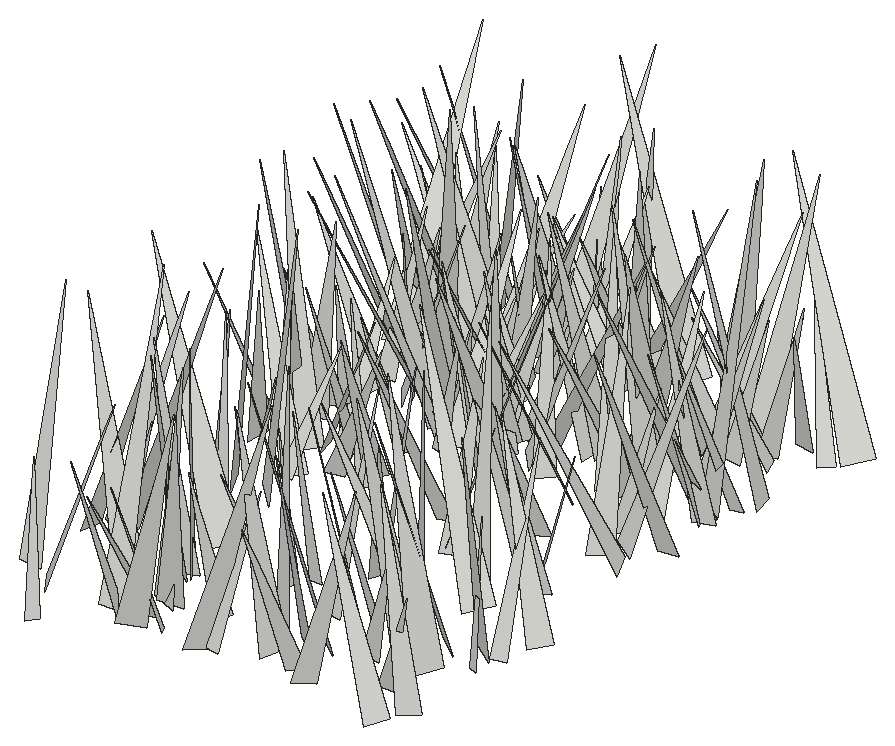
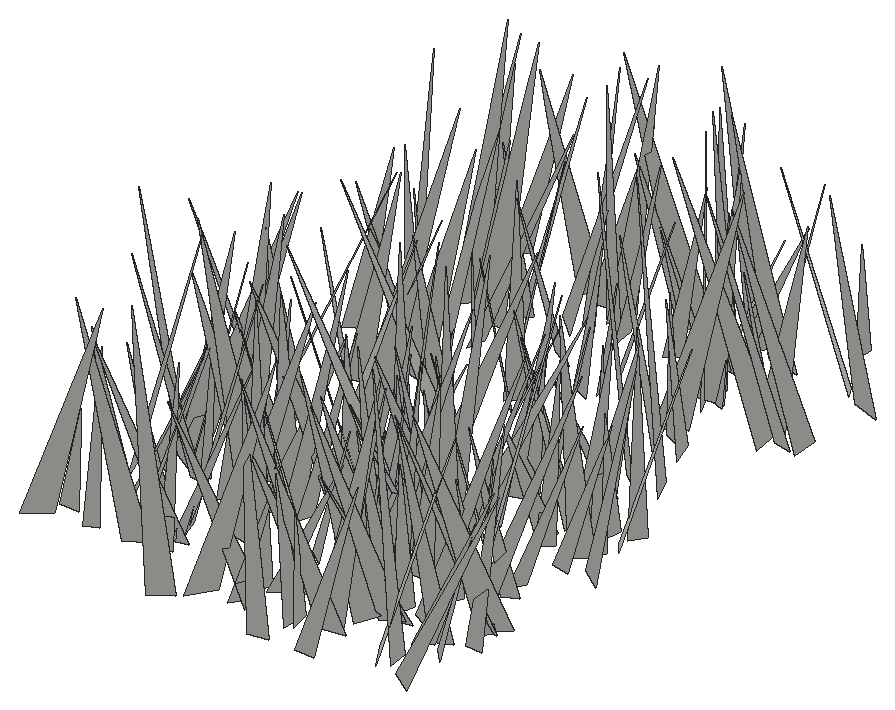
# SketchUp Ruby script. Lengths in inches.
U = 1.inch
M = Sketchup.active_model
def pt(a) = Geom::Point3d.new(a.map { |v| v * U })
def face(e, loops, mat)
  f = e.add_face(loops[0].map { |a| pt(a) })
  loops[1..].each { |l| e.add_face(l.map { |a| pt(a) }).erase! }
  f.material = f.back_material = mat if mat
  f
end
# faces: each face lists its corners as indices into pts; further lists are holes
def faces(e, pts, list, mat = nil) = list.each { |f| face(e, (f[0].is_a?(Array) ? f : [f]).map { |l| l.map { |i| pts[i] } }, mat) }
# xy, xz, yz: faces in a plane at the given z, y or x. An outline is a flat list of corners, or four numbers for a rectangle; further outlines are holes
def ring(l) = l.size == 4 ? [[l[0], l[1]], [l[2], l[1]], [l[2], l[3]], [l[0], l[3]]] : l.each_slice(2).to_a
def flat(e, list, mat, &to3) = list.each { |f| face(e, (f[0].is_a?(Array) ? f : [f]).map { |l| ring(l).map { |u, v| to3.(u, v) } }, mat) }
def xy(e, z, list, mat = nil) = flat(e, list, mat) { |x, y| [x, y, z] }
def xz(e, y, list, mat = nil) = flat(e, list, mat) { |x, z| [x, y, z] }
def yz(e, x, list, mat = nil) = flat(e, list, mat) { |y, z| [x, y, z] }
def lines(e, pts, list) = list.each { |a, b| e.add_line(pt(pts[a]), pt(pts[b])) }
# prism: a flat outline (further loops are holes) pulled along v
def prism(e, loops, v, mat = nil)
  f = face(e, loops, mat); d = Geom::Vector3d.new(v.map { |x| x * U })
  f.pushpull(f.normal.samedirection?(d) ? d.length : -d.length)
end
def box(e, o, s, mat = nil) = prism(e, [[o, [o[0] + s[0], o[1], o[2]], [o[0] + s[0], o[1] + s[1], o[2]], [o[0], o[1] + s[1], o[2]]]], [0, 0, s[2]], mat)
def at(x, y, z, deg = 0) = Geom::Transformation.translation(pt([x, y, z])) * Geom::Transformation.rotation(ORIGIN, Z_AXIS, deg.degrees)
def axes(o, x, y, z) = Geom::Transformation.new([*x, 0, *y, 0, *z, 0, *pt(o).to_a, 1])
def part(name) = M.definitions.add(name)
# library, detail: a bought-in or finely detailed component or shape, given as its bounding box
def library(name, o, s) = part(name).tap { |d| box(d.entities, o, s) }
def detail(e, o, s) = box(e.add_group.entities, o, s)
def put(e, d, t, mat = nil) = e.add_instance(d, t).tap { |i| i.material = mat if mat }
def group(e, t, mat = nil) = e.add_group.tap { |g| g.transformation = t; g.material = mat if mat }.entities
root = M.entities
c1 = part("fur_instance\#9")
p = [[0.8125,0,1.79],[0.67,-0.02,1.48],[0,-0.11,0],[0,0.11,0]]
faces(c1.entities,p,[[0,1,2,3]])
put(root,c1,axes([454.72,184.64,-21.66],[-3.28868,-4.79968,1.75844],[-5.10998,3.14053,-0.98472],[0.13097,2.01112,5.73434]))
put(root,c1,axes([455.49,197.55,-21.66],[-2.53227,-4.93937,0.36335],[-4.86121,2.40071,-1.24381],[-0.94765,0.88376,5.4095]))
put(root,c1,axes([454.7,164.46,-21.66],[1.29784,6.7007,1.25957],[6.74597,-1.44798,0.75208],[-0.98888,-1.08363,6.78367]))
put(root,c1,axes([455.52,181.53,-21.66],[-3.97352,-3.33663,0.47318],[-3.25036,3.98768,0.8243],[0.89005,-0.33346,5.12275]))
put(root,c1,axes([455.72,194.54,-21.66],[-2.9488,-2.48385,0.84804],[-2.61567,2.88641,-0.64107],[0.2167,1.04076,3.80183]))
put(root,c1,axes([456.92,194.2,-21.66],[-4.48303,2.72425,0.35571],[2.72908,4.33728,1.17718],[-0.3165,-1.18832,5.11208]))
put(root,c1,axes([455.09,191.15,-21.66],[-3.2389,7.2108,0.31573],[7.08918,3.2432,-1.34571],[1.35602,0.26802,7.78942]))
put(root,c1,axes([454.82,193.1,-21.66],[-0.80762,-5.18,0.70533],[-5.16495,0.90095,0.70267],[0.80822,0.5814,5.19528]))
put(root,c1,axes([456.91,187.28,-21.66],[-4.89818,0.93846,0.55806],[1.01529,4.8584,0.74127],[0.40164,-0.83642,4.93188]))
put(root,c1,axes([456.51,180.89,-21.66],[-4.24883,1.88722,0.42776],[1.75815,4.19597,-1.04876],[0.80838,0.79335,4.52927]))
put(root,c1,axes([456.4,184.75,-21.66],[-0.08918,-3.86635,0.81214],[-3.84672,-0.10019,-0.89937],[-0.90053,0.81086,3.76135]))
put(root,c1,axes([457.02,168.53,-21.66],[-2.59565,5.50063,1.7013],[5.74289,2.3395,1.19781],[-0.41302,-2.03926,5.96319]))
put(root,c1,axes([457.2,189.25,-21.66],[-2.8111,-5.64649,0.53318],[-5.64839,2.7334,-0.83291],[-0.51273,0.84565,6.25232]))
put(root,c1,axes([458.01,180.9,-21.66],[-6.64184,2.29308,0.28161],[2.23011,6.58737,-1.04152],[0.60342,0.8944,6.94892]))
put(root,c1,axes([457.86,196.35,-21.66],[-5.59539,-3.44886,0.89561],[-3.54081,5.56848,-0.67808],[0.39927,1.05,6.53783]))
put(root,c1,axes([457.09,190.41,-21.66],[-6.10704,-5.17922,1.29191],[-4.99805,6.23748,1.37932],[1.87424,-0.24245,7.88782]))
put(root,c1,axes([455.2,191.6,-21.66],[1.8239,-3.22944,0.77362],[-3.28665,-1.6292,0.94764],[0.47508,1.1273,3.58579]))
put(root,c1,axes([455.38,180.33,-21.66],[4.72712,-1.54603,0.79765],[-1.39638,-4.74943,-0.93014],[-1.03759,-0.65178,4.88576]))
put(root,c1,axes([454.67,168.92,-21.66],[6.22243,-0.20354,0.93497],[-0.30289,-6.25415,0.65425],[-0.90767,0.69164,6.19128]))
put(root,c1,axes([458.11,192.66,-21.66],[-3.1759,-6.57357,0.78945],[-6.61199,3.10387,-0.75436],[-0.34161,1.03711,7.26148]))
put(root,c1,axes([455.91,182.625,-21.66],[4.73789,-1.18845,0.72275],[-0.9672,-4.65874,-1.32025],[-0.99966,-1.12521,4.70287]))
put(root,c1,axes([458.98,178.54,-21.66],[-3.00084,5.06154,0.45444],[5.0055,2.85272,1.2797],[-0.87785,-1.03611,5.74339]))
put(root,c1,axes([455.28,191.36,-21.66],[2.30365,5.6713,0.71156],[5.64313,-2.13475,-1.25489],[0.90837,-1.12069,5.9913]))
put(root,c1,axes([455.6,169.42,-21.66],[2.77668,6.00015,1.42785],[6.14966,-2.57364,-1.14395],[0.47149,-1.76779,6.51177]))
put(root,c1,axes([456.54,188.25,-21.66],[1.07751,-3.9043,2.33703],[-4.53898,-0.75293,0.83488],[0.32078,2.46086,3.96327]))
put(root,c1,axes([456.34,193.5625,-21.66],[-0.43128,5.47544,2.09207],[5.72554,0.84273,-1.02531],[1.25517,-1.9628,5.39585]))
put(root,c1,axes([458.07,160.41,-21.66],[-3.61922,1.27993,0.57976],[1.16278,3.62754,-0.74965],[0.78884,0.52519,3.76496]))
put(root,c1,axes([456.27,183.33,-21.66],[2.75053,-5.09352,1.52718],[-5.31748,-2.64324,0.76119],[-0.02665,1.70616,5.73847]))
put(root,c1,axes([458.72,187.55,-21.66],[-3.32365,-1.7064,1.24939],[-2.04417,3.18881,-1.08271],[0.54234,1.56176,3.57578]))
put(root,c1,axes([457.06,168.4,-21.66],[1.7878,3.1828,1.34143],[3.44443,-1.53093,-0.95817],[0.2561,-1.62848,3.52255]))
put(root,c1,axes([456.9,196.1,-21.66],[6.76883,1.43904,1.95286],[1.74836,-6.90673,-0.9705],[-1.68159,-1.38844,6.85171]))
put(root,c1,axes([460.6,171.4,-21.66],[-6.11884,4.72961,1.11538],[4.85918,5.97068,1.339],[0.0418,-1.7422,7.61686]))
put(root,c1,axes([458.76,172.84,-21.66],[-4.7564,-0.43454,1.78324],[-0.95829,4.81251,-1.3833],[1.56539,1.62573,4.5715]))
put(root,c1,axes([461.03,186.45,-21.66],[-7.48937,-0.81173,0.36322],[-0.84224,7.4632,-0.68756],[0.28542,0.72333,7.50179]))
put(root,c1,axes([457.36,176.08,-21.66],[6.90611,3.10223,2.59996],[3.46907,-7.18559,-0.64093],[-2.08547,-1.6797,7.5437]))
put(root,c1,axes([456.41,163.48,-21.66],[4.70564,3.18962,0.73071],[3.27223,-4.59158,-1.02983],[-0.01227,-1.26267,5.59072]))
put(root,c1,axes([456.45,169.43,-21.66],[7.58645,0.4489,1.20084],[0.2907,-7.62155,1.01257],[-1.24861,0.95304,7.53196]))
put(root,c1,axes([459.54,192.32,-21.66],[-4.60941,2.24833,0.68921],[2.12734,4.63308,-0.88638],[1.00221,0.50623,5.05134]))
put(root,c1,axes([458.27,183.51,-21.66],[3.6116,-2.54944,1.03868],[-2.46348,-3.75778,-0.65768],[-1.22872,0.0404,4.37159]))
put(root,c1,axes([458.75,182.78,-21.66],[-2.94733,3.27814,0.42411],[3.06608,2.92358,-1.29021],[1.23501,0.56503,4.21525]))
put(root,c1,axes([459.77,172.17,-21.66],[0.78619,5.10987,0.99795],[4.99569,-1.02461,1.31074],[-1.46621,-0.75112,5.00108]))
put(root,c1,axes([461.33,186.15,-21.66],[-3.69679,-5.87263,0.02895],[-5.78236,3.6339,-1.23044],[-1.02613,0.67962,6.82936]))
put(root,c1,axes([459.72,182.05,-21.66],[-4.44345,-1.97155,1.25823],[-1.71315,4.58269,1.13072],[1.59225,-0.57131,4.72787]))
put(root,c1,axes([458.6875,178.19,-21.66],[-0.53064,3.51066,0.60828],[3.36851,0.69471,-1.0709],[1.16098,-0.41106,3.38519]))
put(root,c1,axes([462.34,185.2,-21.66],[-6.31151,-2.93767,0.11387],[-2.9284,6.25835,-0.85765],[-0.25951,0.82534,6.90866]))
put(root,c1,axes([458.48,190.38,-21.66],[7.59105,-2.36712,2.02897],[-2.18853,-7.84946,-0.96967],[-2.22043,-0.35586,7.89221]))
put(root,c1,axes([460.87,189.36,-21.66],[-1.86081,5.49202,1.44787],[5.66351,1.67938,0.90859],[-0.42807,-1.65488,5.72707]))
put(root,c1,axes([460.3,163.53,-21.66],[0.64716,8.27924,1.09317],[8.31403,-0.74193,0.69715],[-0.78591,-1.0312,8.27518]))
put(root,c1,axes([460.64,198.27,-21.66],[0.6809,-4.24063,0.83858],[-4.19337,-0.85411,-0.91428],[-1.04966,0.66131,4.19651]))
put(root,c1,axes([458.3,187.27,-21.66],[4.49917,3.28934,0.87918],[3.40387,-4.3112,-1.28935],[0.07989,-1.55853,5.42216]))
put(root,c1,axes([460.62,163.59,-21.66],[-3.9819,-2.09854,0.99873],[-1.89028,4.07705,1.03024],[1.35209,-0.4803,4.38155]))
put(root,c1,axes([461.92,189.72,-21.66],[-6.95078,-0.2098,1.40903],[-0.48679,6.94525,-1.36721],[1.33881,1.43604,6.81821]))
put(root,c1,axes([458.5,181.43,-21.66],[4.5818,0.64032,0.1617],[0.65902,-4.5067,-0.82732],[-0.04299,-0.84188,4.55176]))
put(root,c1,axes([459.15,176.24,-21.66],[-4.14785,-5.45032,3.6874],[-5.74845,5.12259,1.10541],[3.20285,2.13555,6.75935]))
put(root,c1,axes([460.88,168.1875,-21.66],[1.22573,-5.85041,2.29876],[-6.17569,-1.55733,-0.67049],[-1.1715,2.08841,5.93971]))
put(root,c1,axes([459.42,193.3125,-21.66],[-0.94911,6.39885,1.08787],[6.32075,1.1611,-1.31509],[1.4754,-0.85797,6.33377]))
put(root,c1,axes([462.92,189.98,-21.66],[-8.06314,0.9505,0.88883],[1.02226,8.07835,0.63476],[0.80526,-0.7379,8.09412]))
put(root,c1,axes([458.67,193.15,-21.66],[1.67584,3.97009,0.12724],[3.80521,-1.56498,-1.28741],[1.13936,-0.61275,4.1125]))
put(root,c1,axes([460.52,168.18,-21.66],[-2.8459,-6.01928,1.64103],[-5.98512,3.14324,1.14988],[1.76154,0.95508,6.5581]))
put(root,c1,axes([461.53,183.37,-21.66],[0.72019,-3.80208,0.86926],[-3.795,-0.88705,-0.73566],[-0.89965,0.69817,3.79912]))
put(root,c1,axes([462.17,179.63,-21.66],[-0.0394,4.36961,1.02441],[4.32756,-0.23455,1.1669],[-1.18959,-0.99797,4.2111]))
put(root,c1,axes([461.45,195.45,-21.66],[3.35042,-5.0359,1.55374],[-4.92978,-3.64566,-1.18576],[-1.86322,0.59037,5.93123]))
put(root,c1,axes([462.3,164.125,-21.66],[-0.70477,-3.63934,0.22038],[-3.52996,0.62491,-0.96896],[-0.91253,0.39339,3.57807]))
put(root,c1,axes([462.63,193.39,-21.66],[-3.17,-4.98135,1.74667],[-5.27871,2.99065,-1.05117],[-0.00204,2.03858,5.81015]))
put(root,c1,axes([460.64,189.14,-21.66],[-0.56005,-4.94681,0.27227],[-4.82604,0.60667,1.09544],[1.12,0.14049,4.85639]))
put(root,c1,axes([460.34,192.32,-21.66],[2.46707,-3.42013,1.11602],[-3.59628,-2.30764,0.87798],[0.09798,1.4166,4.12467]))
put(root,c1,axes([461.14,187.23,-21.66],[-1.28259,-7.19659,1.19017],[-7.23451,1.40948,0.72639],[0.93233,1.03678,7.27381]))
put(root,c1,axes([459.8,173.39,-21.66],[5.00049,1.26706,0.71261],[1.41038,-4.84715,-1.27832],[-0.35226,-1.4205,4.99762]))
put(root,c1,axes([460.84,168.76,-21.66],[5.57047,2.74276,2.66238],[3.42235,-5.67452,-1.31471],[-1.7025,-2.43273,6.06831]))
put(root,c1,axes([461.21,166.78,-21.66],[2.3019,2.88607,2.09295],[3.52279,-2.224,-0.8077],[-0.54756,-2.17555,3.60219]))
put(root,c1,axes([463.36,163.375,-21.66],[-3.08913,-1.9262,0.20442],[-1.91689,2.98464,-0.84391],[-0.27849,0.82245,3.5413]))
put(root,c1,axes([462.66,196.09,-21.66],[-3.84179,0.25674,0.88435],[-0.00822,3.78425,-1.13434],[0.92083,1.10494,3.67947]))
put(root,c1,axes([460.93,195.9,-21.66],[0.33819,7.69063,1.05021],[7.70297,-0.20312,-0.99305],[0.95553,-1.08446,7.63374]))
put(root,c1,axes([460.35,179.74,-21.66],[2.89103,-3.61881,0.35286],[-3.55779,-2.72252,1.22815],[0.74997,1.03461,4.46604]))
put(root,c1,axes([462.12,192.11,-21.66],[-3.33376,-1.76985,1.3611],[-1.54667,3.5947,0.88593],[1.61021,-0.21143,3.66899]))
put(root,c1,axes([462.88,196.28,-21.66],[-4.76791,1.69378,1.39092],[1.4281,4.92716,-1.10462],[1.66255,0.62512,4.93778]))
put(root,c1,axes([461.76,165.45,-21.66],[2.13967,5.72529,2.72362],[6.33838,-1.99885,-0.77766],[-0.14822,-2.82858,6.06237]))
put(root,c1,axes([462.09,180.71,-21.66],[3.35364,-3.87615,0.32814],[-3.76663,-3.34394,-1.00479],[-0.97195,-0.41544,5.02611]))
put(root,c1,axes([461.46,187.02,-21.66],[0.44835,5.06558,1.88586],[5.29017,-0.02286,-1.19629],[1.10933,-1.93829,4.94267]))
put(root,c1,axes([460.37,193.96,-21.66],[4.49175,-3.99144,0.42922],[-3.97143,-4.32409,1.3497],[0.58618,1.28931,5.8554]))
put(root,c1,axes([464.54,188.46,-21.66],[-2.68226,-4.58353,0.12394],[-4.53778,2.63294,-0.83358],[-0.65781,0.52677,5.24485]))
put(root,c1,axes([461.85,191.2,-21.66],[0.25447,-5.59234,1.88155],[-5.79418,0.11887,1.13692],[1.11444,1.89496,5.48146]))
put(root,c1,axes([461.93,186.69,-21.66],[1.922,-3.18961,0.22781],[-3.1707,-1.86642,0.61867],[0.41494,0.51232,3.67219]))
put(root,c1,axes([463.05,185.25,-21.66],[-2.73527,5.15415,0.70761],[4.98067,2.82527,-1.3261],[1.50298,0.0175,5.68229]))
put(root,c1,axes([462.11,165.52,-21.66],[1.6892,-5.96403,1.00433],[-6.01842,-1.55459,0.89085],[0.59746,1.20222,6.13428]))
put(root,c1,axes([465.25,194.59,-21.66],[-3.7614,2.09395,0.36046],[2.10674,3.58022,1.1859],[-0.27609,-1.20834,4.13841]))
put(root,c1,axes([462.02,193.02,-21.66],[2.06201,-3.51619,0.27094],[-3.44771,-1.94389,1.0117],[0.74186,0.73932,3.94867]))
put(root,c1,axes([461.9,162.84,-21.66],[4.17452,-5.37379,1.20818],[-5.50555,-4.02647,1.11376],[0.16212,1.6352,6.71296]))
put(root,c1,axes([464.62,185.32,-21.66],[2.18952,-4.24382,2.13551],[-4.35668,-2.73133,-0.96101],[-1.89466,1.3763,4.67766]))
put(root,c1,axes([462.91,184.33,-21.66],[0.44262,-3.83329,1.02735],[-3.85493,-0.16968,1.02773],[0.94293,1.1057,3.71938]))
put(root,c1,axes([462.92,187.66,-21.66],[1.90373,-3.64825,0.45227],[-3.65968,-1.83258,0.622],[0.34793,0.68584,4.0678]))
put(root,c1,axes([465.58,186.24,-21.66],[-4.50739,-0.00087,0.31518],[-0.09503,4.31184,-1.34718],[0.30051,1.35052,4.30136]))
put(root,c1,axes([463.1,186.73,-21.66],[1.23248,3.89294,0.26564],[3.83774,-1.15903,-0.82034],[0.70519,-0.49622,4.00013]))
put(root,c1,axes([463.73,193.62,-21.66],[-1.59492,4.69203,0.53683],[4.53057,1.68008,-1.22409],[1.33316,-0.09626,4.80214]))
put(root,c1,axes([463.3,198.36,-21.66],[0.07384,-6.03784,2.03973],[-6.28438,0.27016,1.02718],[1.05955,2.02311,5.95028]))
put(root,c1,axes([465.38,170.51,-21.66],[-3.65849,-0.26653,0.63033],[-0.40108,3.61269,-0.80033],[0.55452,0.85461,3.57982]))
put(root,c1,axes([464.78,166.02,-21.66],[3.15907,-2.58161,1.45094],[-2.40771,-3.47422,-0.93937],[-1.72421,0.12146,3.97014]))
put(root,c1,axes([465.85,190.92,-21.66],[-2.1087,-2.96786,0.97974],[-3.12443,1.97245,-0.74971],[-0.07759,1.23123,3.56269]))
put(root,c1,axes([465.16,187.47,-21.66],[3.57581,-3.48366,1.446],[-3.33217,-3.85124,-1.03819],[-1.76733,0.21279,4.88308]))
put(root,c1,axes([465.68,168.83,-21.66],[-3.61169,-1.5954,0.61372],[-1.41522,3.59542,1.01805],[0.9587,-0.70282,3.81487]))
put(root,c1,axes([467.91,196.77,-21.66],[-7.19785,3.45896,0.52945],[3.49375,7.17168,0.64382],[0.19618,-0.81015,7.95983]))
put(root,c1,axes([466.17,196.42,-21.66],[-3.68845,0.83243,0.84341],[0.99836,3.66829,0.74556],[0.6384,-0.92717,3.70698]))
put(root,c1,axes([465.16,186.97,-21.66],[3.88583,-1.17381,1.38743],[-0.79486,-4.04284,-1.19419],[-1.63432,-0.82466,3.87962]))
put(root,c1,axes([466.03,171.29,-21.66],[-1.43157,-3.77915,1.63266],[-4.11341,1.2436,-0.72817],[-0.16553,1.78,3.97506]))
put(root,c1,axes([467.07,179.57,-21.66],[-0.62326,-5.57048,0.69706],[-5.46922,0.44429,-1.33972],[-1.26641,0.82277,5.44278]))
put(root,c1,axes([464.5,186.88,-21.66],[-0.11814,4.24138,1.60816],[4.31681,0.59918,-1.26317],[1.39308,-1.49704,4.05064]))
put(root,c1,axes([463.92,186.45,-21.66],[7.5502,3.19495,0.69372],[3.12341,-7.56468,0.84526],[-0.96605,0.51231,8.15468]))
put(root,c1,axes([467.69,166.0625,-21.66],[-5.58164,-0.15602,0.84627],[-0.25003,5.60842,-0.61509],[0.82341,0.64537,5.54984]))
put(root,c1,axes([465.31,187.76,-21.66],[3.08965,-1.86478,1.07968],[-2.12915,-2.93231,1.02827],[-0.33144,1.45368,3.45919]))
put(root,c1,axes([465.74,184.63,-21.66],[0.59547,-6.22896,1.95156],[-6.50827,-0.41619,0.65745],[0.50087,1.99748,6.22272]))
put(root,c1,axes([468.1,185.48,-21.66],[-5.05186,2.37101,0.85511],[2.22237,5.09377,-0.9944],[1.18912,0.55319,5.49128]))
put(root,c1,axes([466.09,194.84,-21.66],[6.0824,-3.06076,1.36011],[-2.97573,-6.23245,-0.71791],[-1.53726,-0.04598,6.77115]))
put(root,c1,axes([466.07,163.35,-21.66],[-0.49271,4.25835,1.65602],[4.30491,0.99075,-1.26683],[1.53091,-1.41548,4.0953]))
put(root,c1,axes([467.46,174.58,-21.66],[2.96652,3.66752,1.13191],[3.55325,-3.16507,0.94281],[-1.45132,-0.25254,4.62191]))
put(root,c1,axes([468.52,188.41,-21.66],[-5.18821,0.426,1.12668],[0.56814,5.25845,0.62796],[1.06213,-0.73187,5.16766]))
put(root,c1,axes([465.73,163.03,-21.66],[6.31096,-2.97385,1.65761],[-3.28181,-6.24286,1.29466],[-0.9062,1.89806,6.85536]))
put(root,c1,axes([465.36,196.02,-21.66],[5.25696,-1.00652,0.21452],[-1.02902,-5.15697,1.02054],[-0.01477,1.04274,5.25426]))
put(root,c1,axes([468.82,189.11,-21.66],[-6.42976,0.15301,2.02637],[0.5172,6.6259,1.14077],[1.96522,-1.24316,6.3296]))
put(root,c1,axes([468.62,165.54,-21.66],[2.86323,5.98862,2.41998],[6.20716,-3.28322,0.78076],[-1.78634,-1.80966,6.59182]))
put(root,c1,axes([468.7,164.91,-21.66],[-5.74569,2.33772,2.68731],[2.89131,6.03979,0.92776],[2.08013,-1.9379,6.13328]))
put(root,c1,axes([468.82,175.49,-21.66],[3.80015,2.05854,2.10545],[1.83657,-4.34391,0.93228],[-2.30164,-0.0674,4.22014]))
put(root,c1,axes([468.625,169.34,-21.66],[1.97963,5.14738,0.61551],[5.06452,-2.06097,0.94673],[-1.10678,-0.22402,5.43306]))
put(root,c1,axes([466.72,190.62,-21.66],[4.42426,3.38365,0.88099],[3.49585,-4.30744,-1.01209],[-0.06566,-1.34021,5.47712]))
put(root,c1,axes([468.73,180.44,-21.66],[-4.44854,-2.43941,1.67916],[-2.34276,4.75236,0.69742],[1.81157,0.15557,5.02532]))
put(root,c1,axes([466.5,186.25,-21.66],[4.45392,4.12687,0.87812],[4.21021,-4.26347,-1.31776],[0.27618,-1.55927,5.92722]))
put(root,c1,axes([470.43,166.76,-21.66],[-4.6315,-5.30606,1.24554],[-5.44783,4.55599,-0.84886],[0.16366,1.49838,6.99175]))
put(root,c1,axes([469.26,190.68,-21.66],[2.90611,1.79436,1.69144],[1.585,-3.36196,0.84331],[-1.88904,-0.06039,3.30969]))
put(root,c1,axes([469.91,191.76,-21.66],[0.31088,-6.10314,0.84199],[-6.04835,-0.46277,-1.12122],[-1.17245,0.76905,6.00731]))
put(root,c1,axes([467.91,173.6875,-21.66],[4.2644,-2.86076,0.08373],[-2.8192,-4.22473,-0.76148],[-0.49304,-0.58632,5.07831]))
put(root,c1,axes([466.78,187.35,-21.66],[6.19791,-1.23637,0.25272],[-1.26158,-6.10069,1.0939],[-0.02993,1.12232,6.22464]))
put(root,c1,axes([470.0625,184.83,-21.66],[-3.47678,-4.99975,0.07246],[-4.93171,3.44331,0.95532],[0.82523,-0.48669,6.01439]))
put(root,c1,axes([470.6,188.27,-21.66],[-0.13118,-4.53208,0.33432],[-4.41868,0.04908,-1.06843],[-1.06148,0.35576,4.40629]))
put(root,c1,axes([469.26,177.22,-21.66],[-2.32023,4.26891,1.78267],[4.38145,2.66784,-0.68595],[1.48474,-1.20167,4.81004]))
put(root,c1,axes([469.46,166.38,-21.66],[-2.94569,-5.43055,1.36405],[-5.282,3.20651,1.35919],[1.85796,0.50597,6.02666]))
put(root,c1,axes([470.4375,164.34,-21.66],[1.77342,-4.13167,0.71101],[-4.001,-1.89854,-1.053],[-1.2523,0.21471,4.37115]))
put(root,c1,axes([471.06,186.47,-21.66],[-5.70691,2.72816,1.15825],[2.57005,5.80682,-1.01437],[1.47624,0.43731,6.24361]))
put(root,c1,axes([468.4,178.18,-21.66],[6.55777,3.05775,0.67545],[3.00333,-6.58518,0.65252],[-0.88663,0.30968,7.20614]))
put(root,c1,axes([471.88,193.52,-21.66],[-5.02334,-0.16728,0.55191],[-0.071,4.98153,0.86367],[0.57231,-0.85028,4.95137]))
put(root,c1,axes([470.625,170,-21.66],[-3.85431,-2.63258,1.04926],[-2.43046,3.98156,1.06172],[1.4575,-0.32233,4.54521]))
put(root,c1,axes([471.11,180.98,-21.66],[1.71301,-8.16044,0.92704],[-8.06805,-1.84913,-1.36891],[-1.53583,0.61199,8.22516]))
put(root,c1,axes([472.6,170.74,-21.66],[-6.27523,-0.24227,0.55286],[-0.1392,6.19931,1.13667],[0.58735,-1.11924,6.17618]))
put(root,c1,axes([469.2,198.13,-21.66],[2.15737,-6.51602,1.69287],[-6.69271,-1.88316,1.28061],[0.7294,1.99342,6.74336]))
put(root,c1,axes([472.07,192.4,-21.66],[-5.80555,-2.80529,1.19859],[-2.69051,5.92298,0.83076],[1.43785,-0.24369,6.39405]))
put(root,c1,axes([472.79,166.85,-21.66],[-4.95008,-4.07189,1.35786],[-4.2827,4.82407,-1.14641],[0.2873,1.75371,6.30629]))
put(root,c1,axes([473.85,177.125,-21.66],[-6.46685,-0.99912,0.02995],[-0.985,6.33639,-1.3035],[-0.17003,1.29271,6.41243]))
put(root,c1,axes([473.5,173.95,-21.66],[-6.02819,4.2729,0.70004],[4.32885,5.97346,0.81585],[0.09372,-1.07093,7.34378]))
put(root,c1,axes([473.23,187.01,-21.66],[0.00148,-6.83986,3.17541],[-7.42007,-0.56775,-1.21947],[-1.34516,3.12424,6.73027]))
put(root,c1,axes([472.67,174.95,-21.66],[0.75585,6.87514,1.87347],[7.05211,-0.99202,0.79528],[-1.02238,-1.75986,6.87069]))
put(root,c1,axes([471.7,194.67,-21.66],[-0.45629,-4.37673,0.42276],[-4.25435,0.54685,1.06962],[1.11127,0.29645,4.26847]))
put(root,c1,axes([471.96,186.62,-21.66],[3.81403,-1.87609,0.65313],[-1.66249,-3.78837,-1.17367],[-1.0874,-0.78844,4.08523]))
put(root,c1,axes([470.39,189.54,-21.66],[5.68552,-4.38043,0.51347],[-4.40819,-5.61738,0.88871],[0.14016,1.01677,7.12204]))
put(root,c1,axes([473.71,194.24,-21.66],[-4.5248,-1.88356,0.71077],[-1.69814,4.51006,1.14127],[1.08134,-0.799,4.76646]))
put(root,c1,axes([473.35,168.97,-21.66],[3.66547,-5.8791,2.24711],[-5.89364,-4.11869,-1.16204],[-2.20868,1.23351,6.83002]))
put(root,c1,axes([472.09,189.07,-21.66],[5.27875,-5.42072,0.96709],[-5.29735,-5.36505,-1.15714],[-1.50251,-0.12916,7.47733]))
put(root,c1,axes([471.5,163.56,-21.66],[4.65487,-3.05281,1.35089],[-3.29302,-4.57961,0.99778],[-0.54826,1.58741,5.47649]))
put(root,c1,axes([471.68,193.72,-21.66],[0.68062,5.93772,0.86921],[5.89172,-0.495,-1.23203],[1.14003,-0.98679,5.84823]))
put(root,c1,axes([472.43,167.32,-21.66],[0.98375,-3.96673,0.69714],[-3.91068,-0.76919,1.14174],[0.96305,0.9285,3.92417]))
put(root,c1,axes([476.0625,181.18,-21.66],[-6.15592,-2.89241,0.11132],[-2.84807,6.09927,0.98037],[0.51666,-0.84058,6.73054]))
put(root,c1,axes([474.63,181.45,-21.66],[-5.4201,3.31702,1.28358],[3.06796,5.54385,-1.37151],[1.7994,0.53923,6.20476]))
put(root,c1,axes([473.25,194.88,-21.66],[-1.23701,6.48468,1.94316],[6.59867,1.59608,-1.12573],[1.51147,-1.6609,6.50492]))
put(root,c1,axes([474.5,167.84,-21.66],[-2.85824,2.70123,1.97363],[3.21945,2.92659,0.65696],[0.90938,-1.87078,3.87745]))
put(root,c1,axes([475.5625,192.8,-21.66],[-4.15133,-1.53142,0.10873],[-1.49707,4.10736,0.69206],[0.34034,-0.61232,4.37033]))
put(root,c1,axes([474.75,176.82,-21.66],[1.57492,-4.967,1.49516],[-5.0252,-1.8484,-0.84719],[-1.28605,1.13987,5.14138]))
put(root,c1,axes([474.52,170.37,-21.66],[-3.9391,-6.11846,0.96009],[-6.01065,4.05101,1.1555],[1.49311,0.1661,7.18449]))
put(root,c1,axes([475.28,167.86,-21.66],[-6.5147,3.53544,2.59254],[3.94464,6.75335,0.70282],[1.91322,-1.88542,7.3788]))
put(root,c1,axes([474.13,185.84,-21.66],[-1.65909,5.33475,1.21269],[5.33342,1.85943,-0.88312],[1.21852,-0.87506,5.51654]))
put(root,c1,axes([474,183.55,-21.66],[3.26385,-1.40609,1.47007],[-1.85279,-3.20219,1.05074],[-0.83985,1.59994,3.39496]))
put(root,c1,axes([476.4,162.79,-21.66],[-4.85696,2.92878,0.85344],[3.03677,4.79447,0.82904],[0.29007,-1.15391,5.61075]))
put(root,c1,axes([476.07,187.34,-21.66],[-1.07248,-7.00957,0.36815],[-6.96342,1.01561,-0.94825],[-0.88342,0.50425,7.02746]))
put(root,c1,axes([473.33,178.84,-21.66],[4.06757,1.21437,0.51699],[1.31683,-3.847,-1.32426],[-0.08902,-1.4188,4.03313]))
put(root,c1,axes([473.83,192.02,-21.66],[1.31447,-3.85278,1.5031],[-4.0825,-0.95693,1.11736],[0.66058,1.75255,3.91449]))
put(root,c1,axes([474.52,188.18,-21.66],[-1.23844,-4.00226,0.78585],[-3.84524,1.41955,1.16979],[1.36007,0.36904,4.02286]))
put(root,c1,axes([477.5625,189.74,-21.66],[-7.02647,-2.17808,1.10616],[-2.29777,7.03636,-0.74079],[0.82938,1.04138,7.31892]))
put(root,c1,axes([474.31,194.39,-21.66],[3.53808,2.09554,0.91862],[2.27584,-3.39762,-1.01485],[-0.23603,-1.34836,3.98489]))
put(root,c1,axes([476.51,186.7,-21.66],[0.19192,-5.71021,2.24229],[-6.02696,-0.59408,-0.99702],[-1.14462,2.17066,5.62577]))
put(root,c1,axes([476.96,188.5625,-21.66],[-0.99125,-4.30354,0.98962],[-4.28593,0.69339,-1.27766],[-1.06332,1.21702,4.22737]))
put(root,c1,axes([476.16,186.92,-21.66],[-4.22717,-2.44585,1.01456],[-2.28976,4.33627,0.91336],[1.32985,-0.3083,4.79759]))
put(root,c1,axes([478.47,195.63,-21.66],[-6.09178,4.42452,0.24879],[4.41982,6.03543,0.88707],[-0.32169,-0.86331,7.47659]))
put(root,c1,axes([475.91,187.91,-21.66],[3.67219,7.15908,2.03524],[7.27938,-3.92759,0.68132],[-1.55086,-1.48365,8.01705]))
put(root,c1,axes([476.96,183.51,-21.66],[-0.56263,-5.96411,0.83016],[-5.9756,0.45013,-0.816],[-0.74291,0.89616,5.93475]))
put(root,c1,axes([474.76,165.52,-21.66],[1.46313,-3.34357,0.17988],[-3.25058,-1.37123,0.95187],[0.80348,0.54115,3.52337]))
put(root,c1,axes([477.14,164.24,-21.66],[1.60632,-4.77246,2.92285],[-5.28453,-2.29441,-0.84211],[-1.84207,2.42054,4.96463]))
put(root,c1,axes([477.6,194.34,-21.66],[-1.23895,4.11427,0.01816],[3.97981,1.19363,1.09497],[-1.04341,-0.33255,4.15491]))
put(root,c1,axes([474.86,193.39,-21.66],[3.32524,-3.2763,0.88677],[-3.39381,-3.22791,0.80025],[-0.05063,1.1934,4.59902]))
put(root,c1,axes([474.6875,188.6,-21.66],[2.54446,5.11145,1.43196],[5.2695,-2.24073,-1.36501],[0.64019,-1.87187,5.54418]))
put(root,c1,axes([476.77,169.39,-21.66],[1.67627,3.15128,1.04901],[3.10636,-1.90337,0.75402],[-1.17538,-0.53615,3.48882]))
put(root,c1,axes([477.89,172.97,-21.66],[-4.17135,3.80631,1.04328],[3.93898,4.10999,0.75433],[0.24669,-1.26356,5.59635]))
put(root,c1,axes([475.7,195.11,-21.66],[0.30074,-4.21199,0.28121],[-4.14735,-0.24225,0.80695],[0.78703,0.33293,4.14489]))
put(root,c1,axes([477.17,170.79,-21.66],[0.66443,5.27954,0.01832],[5.19176,-0.65673,0.9642],[-0.95891,0.10252,5.2331]))
put(root,c1,axes([476.15,170.9,-21.66],[-2.86307,-5.78602,1.82095],[-5.78172,3.21211,1.11581],[1.83453,1.09334,6.35847]))
put(root,c1,axes([475.16,182.51,-21.66],[3.14685,5.37097,0.90824],[5.43729,-3.03382,-0.89816],[0.32882,-1.23429,6.15981]))
